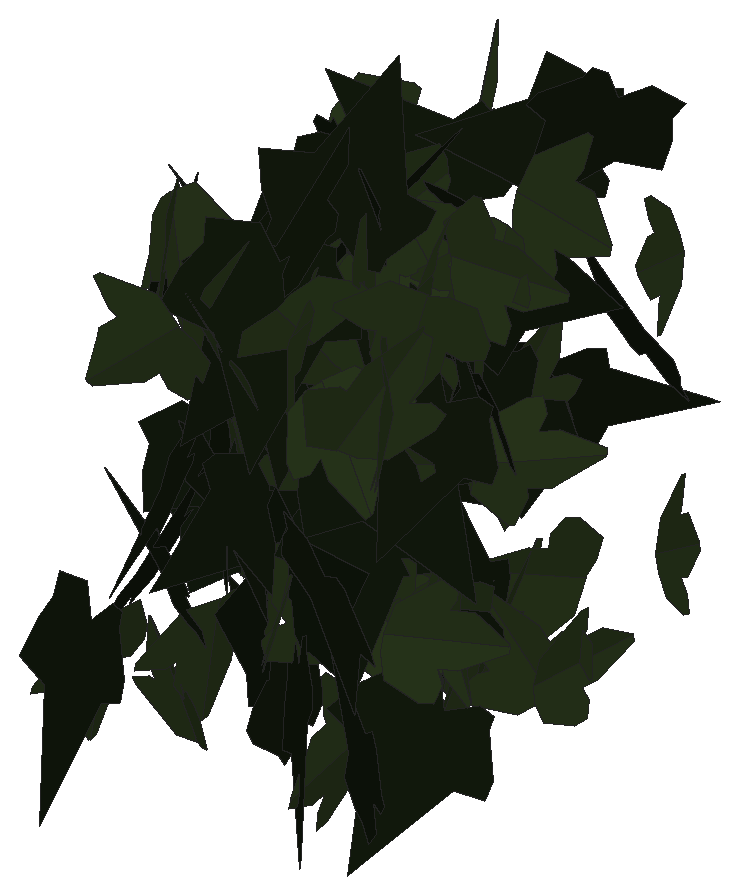
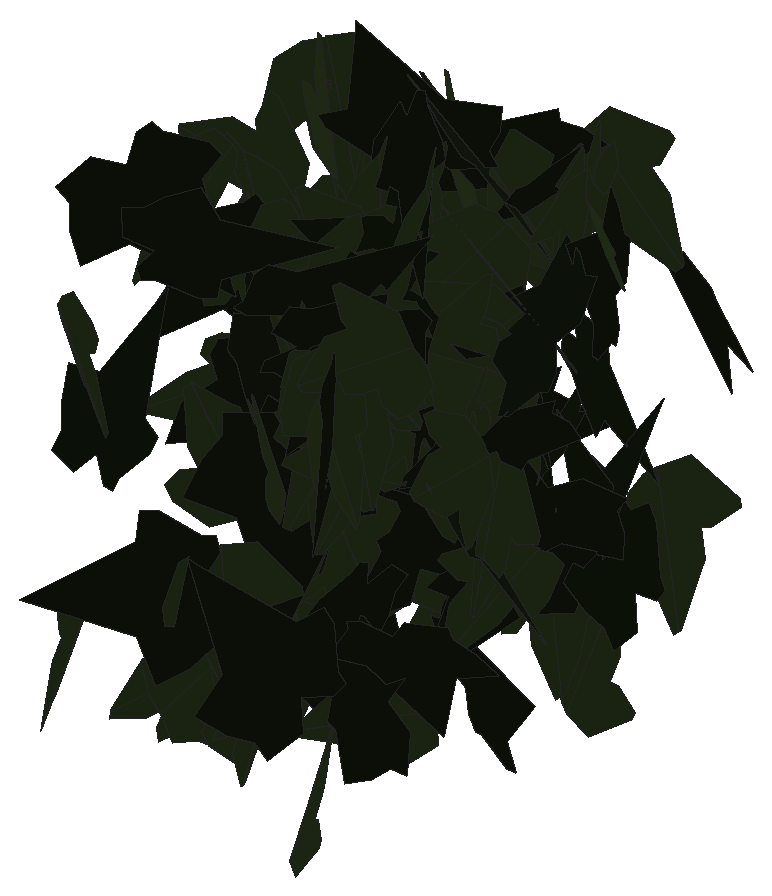
# SketchUp Ruby script. Lengths in inches.
U = 1.inch
M = Sketchup.active_model
def pt(a) = Geom::Point3d.new(a.map { |v| v * U })
def face(e, loops, mat)
  f = e.add_face(loops[0].map { |a| pt(a) })
  loops[1..].each { |l| e.add_face(l.map { |a| pt(a) }).erase! }
  f.material = f.back_material = mat if mat
  f
end
# faces: each face lists its corners as indices into pts; further lists are holes
def faces(e, pts, list, mat = nil) = list.each { |f| face(e, (f[0].is_a?(Array) ? f : [f]).map { |l| l.map { |i| pts[i] } }, mat) }
# xy, xz, yz: faces in a plane at the given z, y or x. An outline is a flat list of corners, or four numbers for a rectangle; further outlines are holes
def ring(l) = l.size == 4 ? [[l[0], l[1]], [l[2], l[1]], [l[2], l[3]], [l[0], l[3]]] : l.each_slice(2).to_a
def flat(e, list, mat, &to3) = list.each { |f| face(e, (f[0].is_a?(Array) ? f : [f]).map { |l| ring(l).map { |u, v| to3.(u, v) } }, mat) }
def xy(e, z, list, mat = nil) = flat(e, list, mat) { |x, y| [x, y, z] }
def xz(e, y, list, mat = nil) = flat(e, list, mat) { |x, z| [x, y, z] }
def yz(e, x, list, mat = nil) = flat(e, list, mat) { |y, z| [x, y, z] }
def lines(e, pts, list) = list.each { |a, b| e.add_line(pt(pts[a]), pt(pts[b])) }
# prism: a flat outline (further loops are holes) pulled along v
def prism(e, loops, v, mat = nil)
  f = face(e, loops, mat); d = Geom::Vector3d.new(v.map { |x| x * U })
  f.pushpull(f.normal.samedirection?(d) ? d.length : -d.length)
end
def box(e, o, s, mat = nil) = prism(e, [[o, [o[0] + s[0], o[1], o[2]], [o[0] + s[0], o[1] + s[1], o[2]], [o[0], o[1] + s[1], o[2]]]], [0, 0, s[2]], mat)
def at(x, y, z, deg = 0) = Geom::Transformation.translation(pt([x, y, z])) * Geom::Transformation.rotation(ORIGIN, Z_AXIS, deg.degrees)
def axes(o, x, y, z) = Geom::Transformation.new([*x, 0, *y, 0, *z, 0, *pt(o).to_a, 1])
def part(name) = M.definitions.add(name)
# library, detail: a bought-in or finely detailed component or shape, given as its bounding box
def library(name, o, s) = part(name).tap { |d| box(d.entities, o, s) }
def detail(e, o, s) = box(e.add_group.entities, o, s)
def put(e, d, t, mat = nil) = e.add_instance(d, t).tap { |i| i.material = mat if mat }
def group(e, t, mat = nil) = e.add_group.tap { |g| g.transformation = t; g.material = mat if mat }.entities
root = M.entities
M.materials.add("efeu1").color = [18, 25, 13]
M.materials.add("efeu2").color = [43, 57, 29]
c1 = part("ivyleaf_10")
p = [[0,0.5,-0.03],[-0.0625,2.02,-0.43],[-0.19,2.01,-0.46],[-0.54,1.05,-0.29],[-0.52,0.625,-0.18],[-0.83,0.76,-0.28],
  [-1.16,0.64,-0.33],[-1.15,0.33,-0.24],[-0.77,-0.39,0.02],[-0.3,-0.51,0.16],[0.04,-0.48,0.23],[-0.02,2.01,-0.4375],
  [-0.06,2.01,-0.43],[0.04,-0.49,0.23],[0.67,-0.49,0.14],[1.38,0.36,-0.2],[1.375,0.51,-0.24],[0.81,0.65,-0.19],
  [0.62,0.59,-0.15],[0.6,1.09,-0.28],[0.5,1.23,-0.31]]
faces(c1.entities,p,[[0,1,2,3,4,5,6,7,8,9,10],[11,12,0,13,14,15,16,17,18,19,20]],"efeu2")
c2 = part("ivyleaf_9")
p = [[1.54,2.16,1.25],[1.36,2.04,1.19],[-0.21,0.99,0.68],[-0.71,1.11,0.82],[-0.85,0.86,0.67],[-0.8,0.17,0.21],
  [-0.9,-0.01,0.1],[-0.67,-0.16,-0.02],[-0.08,-0.08,-0.05],[-0.03,-0.6,-0.4],[0.65,-0.88,-0.66],[0.83,-0.6,-0.49],
  [1.29,-0.42,-0.43],[1.8125,-0.07,-0.26],[1.21,0.44,0.15]]
faces(c2.entities,p,[[0,1,2,3,4,5,6,7,8,9,10,11,12,13,14]],"efeu1")
put(root,c1,axes([532.14,136.34,169.07],[-0.45587,0.27288,-0.53992],[0.47143,-0.26343,-0.53118],[-0.37912,-0.6557,-0.01129]))
put(root,c1,axes([532.6,135.1,167.98],[0.05892,-0.64867,-0.52976],[-0.0226,0.52964,-0.65104],[0.8372,0.05995,0.0197]))
put(root,c2,axes([532,134.74,170.28],[0.46444,-0.54922,0.45596],[0.31026,-0.33458,-0.71905],[0.64286,0.55826,0.01763]))
put(root,c2,axes([532.72,132.56,169.79],[0.08276,-0.1459,0.76396],[0.16332,0.7544,0.12638],[-0.76042,0.14615,0.11029]))
put(root,c2,axes([532.37,132.63,165.53],[0.10503,0.7706,0.41637],[-0.05413,-0.41284,0.77773],[0.87422,-0.11814,-0.00187]))
put(root,c2,axes([532.68,137.18,166.59],[-0.58871,-0.4398,-0.24676],[0.19442,0.15205,-0.73483],[0.46531,-0.61997,-0.00517]))
put(root,c2,axes([532.27,139.82,167.11],[0.48732,0.59527,-0.0229],[0.01412,0.01804,0.7693],[0.59554,-0.48753,0.0005]))
put(root,c2,axes([533.14,135.46,167.74],[-0.63921,0.41352,-0.04166],[0.03445,-0.02344,-0.76131],[-0.41418,-0.64014,0.00097]))
put(root,c2,axes([532.71,135.3,168.79],[-0.16537,-0.7849,-0.26819],[0.03211,0.26721,-0.80182],[0.82884,-0.16695,-0.02244]))
put(root,c1,axes([532.66,134.64,166.57],[0.22438,0.59132,0.48602],[0.18814,0.44833,-0.63232],[-0.74195,0.29251,-0.01336]))
put(root,c1,axes([533.17,132.67,163.73],[-0.70067,0.30852,-0.17835],[-0.16614,0.06525,0.76556],[0.31526,0.72007,0.00704]))
put(root,c2,axes([532.63,134.1,167.49],[-0.22629,-0.50109,-0.65626],[0.36018,0.55241,-0.54598],[0.743,-0.4204,0.0648]))
put(root,c1,axes([532.98,139.4,169.94],[0.55214,-0.5034,0.20296],[-0.14896,0.13786,0.74718],[-0.52194,-0.57188,0.00146]))
put(root,c1,axes([532.66,132.95,171.26],[0.43565,-0.38142,0.66927],[0.48674,-0.45965,-0.57879],[0.59707,0.65302,-0.01649]))
put(root,c1,axes([532.97,132.79,171.45],[-0.03904,0.78379,-0.08296],[-0.00243,-0.08318,-0.78474],[-0.78817,-0.03857,0.00653]))
put(root,c1,axes([533.18,130.91,165.76],[-0.11096,-0.87133,-0.02569],[0.00652,0.02507,-0.87836],[0.87168,-0.11111,0.0033]))
put(root,c2,axes([533.25,132.52,165.84],[0.31121,-0.6475,0.32196],[-0.1367,0.29151,0.7184],[-0.71009,-0.3399,0.0028]))
put(root,c2,axes([533.46,137.47,170.09],[0.04667,0.02468,-0.80853],[-0.71578,0.37851,-0.02976],[0.3768,0.71598,0.0436]))
put(root,c1,axes([532.83,135.44,168.63],[0.1385,-0.21962,0.72972],[0.47241,-0.55722,-0.25737],[0.59796,0.4911,0.03431]))
put(root,c2,axes([532.82,134.375,166.43],[0.09054,-0.55616,-0.63736],[0.06071,0.64362,-0.553],[0.84372,0.01337,0.10819]))
put(root,c1,axes([533.09,135.49,169.93],[0.16803,-0.43379,0.74037],[0.23468,-0.70244,-0.46483],[0.82538,0.28804,-0.01856]))
put(root,c1,axes([532.64,137.3,170.99],[0.38534,0.09768,0.6969],[0.63664,0.29015,-0.39269],[-0.29984,0.7416,0.06185]))
put(root,c1,axes([533.25,137.875,169.92],[0.14076,-0.72035,0.1083],[0.01844,-0.10674,-0.73397],[0.72821,0.14194,-0.00235]))
put(root,c1,axes([533.73,136.43,170.05],[0.09018,-0.02225,-0.77113],[-0.59812,0.48833,-0.08404],[0.48723,0.60358,0.03956]))
put(root,c1,axes([533.65,137.07,170.15],[-0.78902,-0.18181,0.3115],[-0.30256,-0.07418,-0.80968],[0.19632,-0.84503,0.00406]))
put(root,c1,axes([532.99,133.98,168.16],[-0.15174,0.09264,-0.72431],[0.40151,-0.60734,-0.16179],[-0.60992,-0.42285,0.07369]))
put(root,c1,axes([534.04,131.15,170.75],[-0.53977,-0.16948,0.65309],[-0.62501,-0.18951,-0.56574],[0.2542,-0.82581,-0.00421]))
put(root,c2,axes([533.12,133.49,167.77],[-0.11876,-0.07689,-0.80535],[0.79433,-0.16548,-0.10134],[-0.15346,-0.79707,0.09872]))
put(root,c1,axes([533.65,132.73,165.43],[-0.20314,-0.85894,-0.02665],[0.00816,0.02546,-0.88263],[0.85932,-0.20329,0.00208]))
put(root,c2,axes([533.9375,133.24,169.74],[-0.83008,0.44308,-0.2176],[-0.19452,0.09766,0.94092],[0.45368,0.85255,0.00531]))
put(root,c2,axes([533.79,131.9,168.32],[-0.58444,0.3954,-0.37179],[0.313,-0.2008,-0.70558],[-0.44339,-0.66293,-0.00803]))
put(root,c1,axes([533.23,134.3,169.89],[0.40623,0.38699,0.6006],[0.44259,0.40606,-0.56101],[-0.56089,0.60071,-0.0077]))
put(root,c2,axes([533.22,133.46,167.28],[0.35087,-0.69906,0.30878],[0.13658,-0.27694,-0.78217],[0.75192,0.37651,-0.00201]))
put(root,c2,axes([534.27,133.67,163.79],[-0.09909,0.13593,0.84531],[-0.45861,0.71015,-0.16795],[-0.72298,-0.4691,-0.00932]))
put(root,c1,axes([533.6,136.38,170.55],[0.11523,-0.34935,0.67031],[0.26244,-0.61739,-0.36688],[0.70887,0.28536,0.02686]))
put(root,c2,axes([533.64,136.67,166.78],[0.25707,-0.26263,-0.66624],[-0.3154,0.59399,-0.35585],[0.64293,0.3964,0.09182]))
put(root,c1,axes([533.26,136.29,164.9],[0.15705,0.12742,0.73398],[0.57256,0.45924,-0.20224],[-0.47659,0.59371,-0.00109]))
put(root,c1,axes([533.18,134.25,169],[0.22204,0.02958,-0.80727],[0.80451,0.06762,0.22376],[0.07305,-0.83452,-0.01049]))
put(root,c2,axes([533.65,136.27,170.75],[0.68589,0.33674,-0.046],[-0.0464,-0.00986,-0.764],[-0.33668,0.68736,0.01158]))
put(root,c1,axes([533.64,134.09,170.85],[-0.32305,-0.34149,-0.58795],[0.41222,0.4193,-0.47003],[0.54072,-0.52368,0.00705]))
put(root,c1,axes([533.67,136.53,168.82],[0.26681,0.7102,0.31257],[0.09965,0.29643,-0.7586],[-0.76951,0.28463,0.01014]))
put(root,c2,axes([533.22,136.79,165.33],[0.3646,-0.02777,-0.73107],[0.67272,0.33375,0.32282],[0.28753,-0.74565,0.17172]))
put(root,c1,axes([533.87,138.46,166],[-0.11314,0.72862,0.06154],[-0.02165,0.05891,-0.73725],[-0.73089,-0.11453,0.01231]))
put(root,c2,axes([534.45,136.9,170.28],[-0.59771,-0.28263,0.57223],[-0.49646,-0.28678,-0.6602],[0.40107,-0.77618,0.03556]))
put(root,c2,axes([533.84,134.4,169.65],[-0.21346,-0.83532,-0.06765],[0.009,0.06753,-0.86213],[0.83801,-0.2135,-0.00798]))
put(root,c1,axes([534.39,136.73,169.54],[-0.08384,-0.08596,0.86544],[-0.32257,-0.80437,-0.11114],[0.80767,-0.33018,0.04545]))
put(root,c1,axes([534.07,136.45,169.05],[-0.44726,-0.49721,-0.40098],[0.26154,0.30404,-0.66873],[0.58275,-0.51806,-0.00762]))
put(root,c1,axes([534.27,137.14,163.09],[-0.49153,0.57496,0.06376],[0.02107,-0.06582,0.75595],[0.5781,0.49126,0.02666]))
put(root,c1,axes([534.06,134.89,171.8125],[-0.07921,0.63149,-0.46442],[0.07105,-0.45908,-0.63634],[-0.78065,-0.10586,-0.0108]))
put(root,c2,axes([534.72,136.84,170.67],[-0.59738,-0.60988,-0.19757],[-0.10545,-0.17289,0.85254],[-0.63235,0.60498,0.04447]))
put(root,c2,axes([534.25,133.11,167.43],[0.07929,-0.18932,-0.73874],[0.21268,-0.70776,0.20421],[-0.73235,-0.22604,-0.02068]))
put(root,c1,axes([534.17,132.9,170.99],[0.23251,-0.75546,0.49666],[0.1685,-0.46763,-0.79018],[0.88826,0.28646,0.01989]))
put(root,c1,axes([534.55,131.97,169.67],[-0.71212,0.22483,-0.27772],[-0.28016,0.03304,0.74513],[0.22178,0.76365,0.04953]))
put(root,c1,axes([534.32,134.08,167.42],[0.07624,-0.55451,0.6336],[0.07554,-0.62912,-0.55968],[0.83859,0.10708,-0.00719]))
put(root,c2,axes([534.19,134.78,170.4],[-0.12773,0.81804,-0.20601],[-0.0636,0.19842,0.82736],[0.84118,0.13922,0.03128]))
put(root,c2,axes([534.27,133.25,170.33],[-0.19178,-0.75154,0.58031],[-0.15693,-0.5588,-0.77555],[0.93645,-0.24756,-0.01112]))
put(root,c2,axes([534.08,134.2,167.95],[-0.328,-0.47585,-0.61472],[0.33892,0.51292,-0.57789],[0.69961,-0.47157,-0.00825]))
put(root,c1,axes([534.55,136.4,170.93],[0.07359,0.19096,-0.7618],[-0.26267,-0.71509,-0.20462],[-0.74015,0.27277,-0.00313]))
put(root,c2,axes([534.34,132.95,165.41],[-0.04446,0.00443,0.82284],[-0.12414,-0.81465,-0.00232],[0.81344,-0.12408,0.04462]))
put(root,c1,axes([534.63,132.94,166.08],[0.46899,-0.61779,-0.19979],[-0.1207,0.15921,-0.77564],[0.63797,0.48428,0.00012]))
put(root,c2,axes([535.03,133.39,172.22],[-0.77593,0.48403,0.02133],[-0.0181,0.01128,-0.91452],[-0.48416,-0.77614,0.00001]))
put(root,c2,axes([534.84,134.25,172.33],[0.36742,0.04049,-0.70012],[-0.69877,-0.04581,-0.36936],[-0.0594,0.78935,0.01447]))
put(root,c1,axes([535.04,135.42,170.54],[-0.08327,-0.26911,0.71982],[-0.24796,-0.67591,-0.28138],[0.72738,-0.26122,-0.01351]))
put(root,c2,axes([534.9375,136.52,168.3],[0.45342,0.6461,-0.32428],[-0.19752,-0.25749,-0.78922],[-0.6954,0.49441,0.01273]))
put(root,c1,axes([535.05,133.75,165.41],[-0.52058,-0.5539,-0.47104],[-0.32442,-0.34152,0.76013],[-0.65072,0.61339,-0.00213]))
put(root,c1,axes([534.99,137.95,167.1],[-0.4535,-0.59208,0.02958],[-0.01469,-0.02601,-0.74579],[0.59264,-0.45372,0.00415]))
put(root,c2,axes([534.51,134.48,165.95],[0.67737,0.39988,0.1042],[-0.09007,-0.0524,0.7866],[0.4033,-0.68333,0.00066]))
put(root,c2,axes([534.61,134.18,169.94],[0.08757,-0.81995,-0.11019],[-0.01387,0.10933,-0.82461],[0.82721,0.08864,-0.00216]))
put(root,c2,axes([534.77,132.75,171.34],[-0.39049,-0.86408,-0.18766],[0.0765,0.17136,-0.94821],[0.8809,-0.39791,-0.00084]))
put(root,c1,axes([534.88,135.51,166.6],[0.19312,0.72146,-0.35683],[-0.09016,-0.34526,-0.74685],[-0.79981,0.21312,-0.00196]))
put(root,c2,axes([534.91,128.4,167.64],[-0.75561,0.002,-0.59826],[0.59821,-0.01008,-0.75558],[-0.00782,-0.96372,0.00666]))
put(root,c2,axes([535.24,135.42,166.57],[0.05106,-0.53417,0.58587],[-0.04226,0.58442,0.53653],[-0.79171,-0.06565,0.00915]))
put(root,c1,axes([535.29,136.24,168.16],[-0.72604,-0.4408,0.22937],[-0.19844,-0.11512,-0.84936],[0.45557,-0.75265,-0.00442]))
put(root,c2,axes([535.54,134.89,169.3125],[-0.26814,-0.72491,-0.50906],[-0.16215,-0.48271,0.77281],[-0.87083,0.3131,0.01285]))
put(root,c2,axes([535.13,133.7,171.68],[-0.6843,0.01154,0.54128],[0.54125,-0.00582,0.68439],[0.01266,0.87248,-0.00259]))
put(root,c1,axes([535.91,134.56,166.09],[-0.34982,-0.1313,-0.77141],[-0.71853,-0.28073,0.37362],[-0.30989,0.79915,0.00451]))
put(root,c1,axes([535.28,132.45,170.83],[-0.438,-0.585,-0.51962],[0.32553,0.40526,-0.73066],[0.71152,-0.54553,0.01442]))
put(root,c2,axes([534.87,133,166.08],[-0.0313,0.01978,0.9289],[0.53375,-0.76038,0.03418],[0.7605,0.53447,0.01425]))
put(root,c2,axes([535.08,132.82,165.02],[-0.31396,0.07614,-0.87026],[0.8543,-0.16647,-0.32277],[-0.18254,-0.91006,-0.01376]))
put(root,c1,axes([534.97,135.13,170.85],[0.35475,0.17542,0.63125],[0.53678,0.33377,-0.39441],[-0.37566,0.64259,0.03254]))
put(root,c2,axes([535.3,133.95,167.05],[-0.12324,-0.77998,-0.09236],[0.01707,0.09081,-0.78966],[0.78525,-0.12439,0.00266]))
put(root,c1,axes([535.29,133.58,163.64],[-0.06176,0.05224,0.89195],[0.40295,-0.79637,0.07454],[0.79746,0.40644,0.03141]))
put(root,c1,axes([535.14,132.57,170.36],[0.26699,-0.50082,-0.66025],[0.37738,-0.54409,0.56532],[-0.73779,-0.45954,0.05023]))
put(root,c1,axes([535.44,134.16,171.43],[-0.05693,0.7349,-0.30371],[0.02755,-0.30248,-0.73709],[-0.7947,-0.06313,-0.0038]))
put(root,c2,axes([536.15,137.76,171.52],[-0.41531,-0.05704,0.67023],[-0.66217,-0.10386,-0.41915],[0.1183,-0.7816,0.00678]))
put(root,c2,axes([535.17,138.33,167.0625],[0.16065,0.36443,-0.67271],[0.2639,0.6188,0.39825],[0.71813,-0.30893,0.00414]))
put(root,c2,axes([535.23,136.14,167.74],[0.10476,-0.40209,0.66671],[0.25063,-0.6195,-0.41299],[0.73713,0.26777,0.04567]))
put(root,c1,axes([535.71,136.49,164.09],[0.20872,-0.7203,0.22222],[-0.06303,0.21309,0.74993],[-0.75116,-0.21803,-0.00118]))
put(root,c1,axes([535.83,134.76,165.75],[0.46603,-0.61961,0.37531],[-0.22573,0.29984,0.77531],[-0.68835,-0.51782,-0.00015]))
put(root,c1,axes([535.71,136.73,167.71],[-0.15338,-0.74678,0.22942],[0.05168,0.22359,0.76235],[-0.77951,0.16176,0.00539]))
put(root,c1,axes([536.04,137.51,164.83],[-0.15647,-0.28352,-0.80973],[-0.36787,-0.72142,0.32368],[-0.77507,0.39964,0.00984]))
put(root,c1,axes([535.88,135.35,163.98],[0.29623,-0.6146,0.41791],[-0.18649,0.37403,0.68225],[-0.71945,-0.35001,-0.00477]))
put(root,c1,axes([536.03,135.03,165.53],[-0.21883,-0.68094,0.3041],[-0.08812,-0.2911,-0.71522],[0.74053,-0.23586,0.00475]))
put(root,c2,axes([535.91,136.2,169.87],[-0.42258,0.31213,-0.57778],[0.45182,-0.36042,-0.52515],[-0.47657,-0.61846,0.01445]))
put(root,c1,axes([535.3,134.21,165.59],[0.22927,0.05961,0.75663],[0.73438,0.18218,-0.23688],[-0.19167,0.76933,-0.00253]))
put(root,c1,axes([535.64,135.65,165.27],[0.24874,-0.25723,0.69894],[0.48015,-0.50792,-0.35781],[0.56933,0.54075,-0.0036]))
put(root,c2,axes([536.18,135.29,165.09],[-0.16177,-0.64486,0.47479],[0.19441,0.43827,0.66149],[-0.77684,0.24397,0.06667]))
put(root,c1,axes([536.3125,135.61,170.65],[-0.4555,-0.60752,0.21564],[-0.12299,-0.17729,-0.75928],[0.63282,-0.47175,0.00765]))
put(root,c2,axes([536.34,135.09,169.17],[0.49649,-0.0131,-0.63003],[-0.63001,0.00724,-0.49663],[0.01379,0.80211,-0.00581]))
put(root,c1,axes([536.49,136.37,163.89],[-0.58936,-0.44573,-0.38986],[-0.3139,-0.23124,0.73891],[-0.50212,0.66772,-0.00435]))
put(root,c1,axes([535.76,133.11,168.45],[-0.34164,-0.02507,0.77516],[0.77031,0.08746,0.34233],[-0.09013,0.84258,-0.01247]))
put(root,c1,axes([536.17,132.21,169.85],[0.3051,0.71883,0.224],[0.09395,0.20346,-0.78087],[-0.74704,0.31916,-0.00672]))
put(root,c1,axes([535.98,135.61,169.81],[0.22959,-0.41364,-0.62472],[0.39189,-0.49059,0.46886],[-0.63859,-0.44978,0.06313]))
put(root,c2,axes([536.73,137.71,172.49],[0.05138,0.35987,-0.70654],[-0.09846,-0.69964,-0.36352],[-0.78677,0.11105,-0.00064]))
put(root,c2,axes([536.64,135.86,168.54],[0.01371,-0.25941,-0.85154],[0.18204,-0.83282,0.25664],[-0.87136,-0.17807,0.04022]))
put(root,c2,axes([536.43,135.51,170.58],[0.14074,0.01105,-0.78214],[-0.22913,0.76043,-0.03049],[0.74791,0.23088,0.13784]))
put(root,c2,axes([536.82,133.73,164.58],[-0.70179,-0.49269,-0.06541],[0.05326,0.03797,-0.85747],[0.49415,-0.7038,-0.00047]))
put(root,c2,axes([536.32,132.93,169.26],[-0.0092,-0.64966,-0.7024],[0.17346,0.68965,-0.64015],[0.94092,-0.13349,0.11114]))
put(root,c1,axes([536.27,134.41,165.71],[0.32242,-0.083,0.65377],[0.6214,-0.20407,-0.33236],[0.21945,0.6998,-0.01938]))
put(root,c2,axes([536.89,138.16,168.46],[0.53004,-0.48981,0.33141],[-0.23384,0.23519,0.72159],[-0.5432,-0.5792,0.01275]))
put(root,c1,axes([536.75,135.08,171.31],[0.72246,-0.22511,0.02698],[0.02597,-0.00737,-0.75672],[0.22523,0.72292,0.00069]))
put(root,c1,axes([536.5,133.86,171.19],[0.17554,-0.41955,-0.66535],[0.30542,-0.59187,0.4538],[-0.72487,-0.35099,0.03007]))
put(root,c1,axes([536.83,135.95,171.68],[-0.08992,0.56013,0.64711],[-0.0854,0.64156,-0.56719],[-0.85159,-0.12349,-0.01145]))
put(root,c1,axes([536.72,132.1,169.8],[-0.31963,-0.74599,0.40367],[0.16045,0.37041,0.81158],[-0.83289,0.35763,0.00143]))
put(root,c2,axes([537.09,131.89,164.24],[0.1056,-0.58066,0.51564],[-0.00733,0.51962,0.58664],[-0.77653,-0.08387,0.06458]))
put(root,c2,axes([536.9375,133.67,169.5],[-0.35426,-0.71717,0.1147],[-0.04371,-0.10633,-0.79986],[0.72497,-0.35686,0.00782]))
put(root,c1,axes([536.99,136.14,164.18],[0.08919,-0.04022,0.75271],[-0.12126,0.74732,0.0543],[-0.74396,-0.12662,0.08138]))
put(root,c1,axes([537.32,138.18,170.09],[0.33739,-0.35819,-0.59038],[-0.40589,0.42872,-0.49207],[0.55866,0.52781,-0.00096]))
put(root,c2,axes([536.52,131.6,167.55],[0.25976,-0.66612,0.54837],[0.20581,-0.50832,-0.71495],[0.8379,0.33136,0.00561]))
put(root,c1,axes([536.87,133.07,166.1],[0.08216,0.20169,0.73887],[0.15388,0.72361,-0.21463],[-0.75028,0.1705,0.03689]))
put(root,c1,axes([537.37,132.71,171.56],[-0.70855,-0.45588,0.23631],[-0.19323,-0.13639,-0.84248],[0.47575,-0.73436,0.00977]))
put(root,c1,axes([537.4,138.09,165.45],[-0.18316,0.23512,0.70547],[-0.41245,0.57244,-0.29787],[-0.61876,-0.45117,-0.01028]))
put(root,c1,axes([536.71,132.8,169.97],[0.09159,-0.07272,0.94033],[0.67068,-0.65921,-0.11631],[0.6631,0.6768,-0.01225]))
put(root,c1,axes([536.52,134.82,171.09],[-0.13629,-0.0007,0.85387],[0.84141,0.14707,0.13442],[-0.14534,0.85208,-0.0225]))
put(root,c1,axes([536.93,134.97,168.14],[-0.03854,-0.13485,-0.74442],[0.51562,0.54077,-0.12466],[0.55361,-0.51305,0.06428]))
